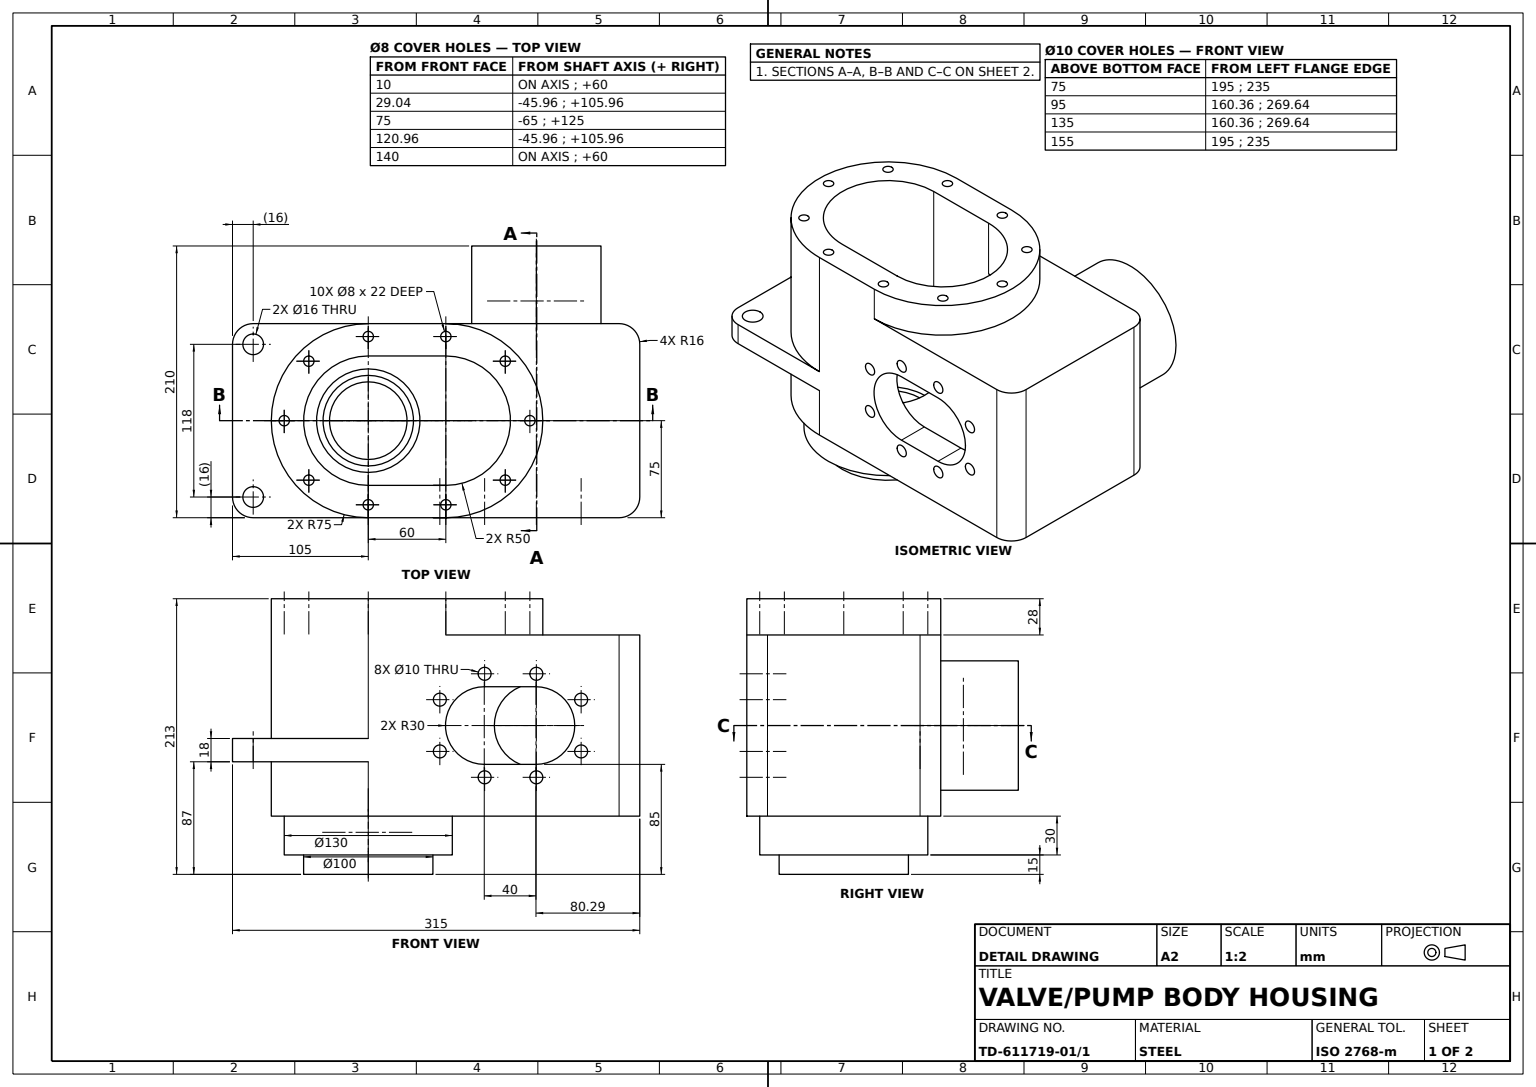
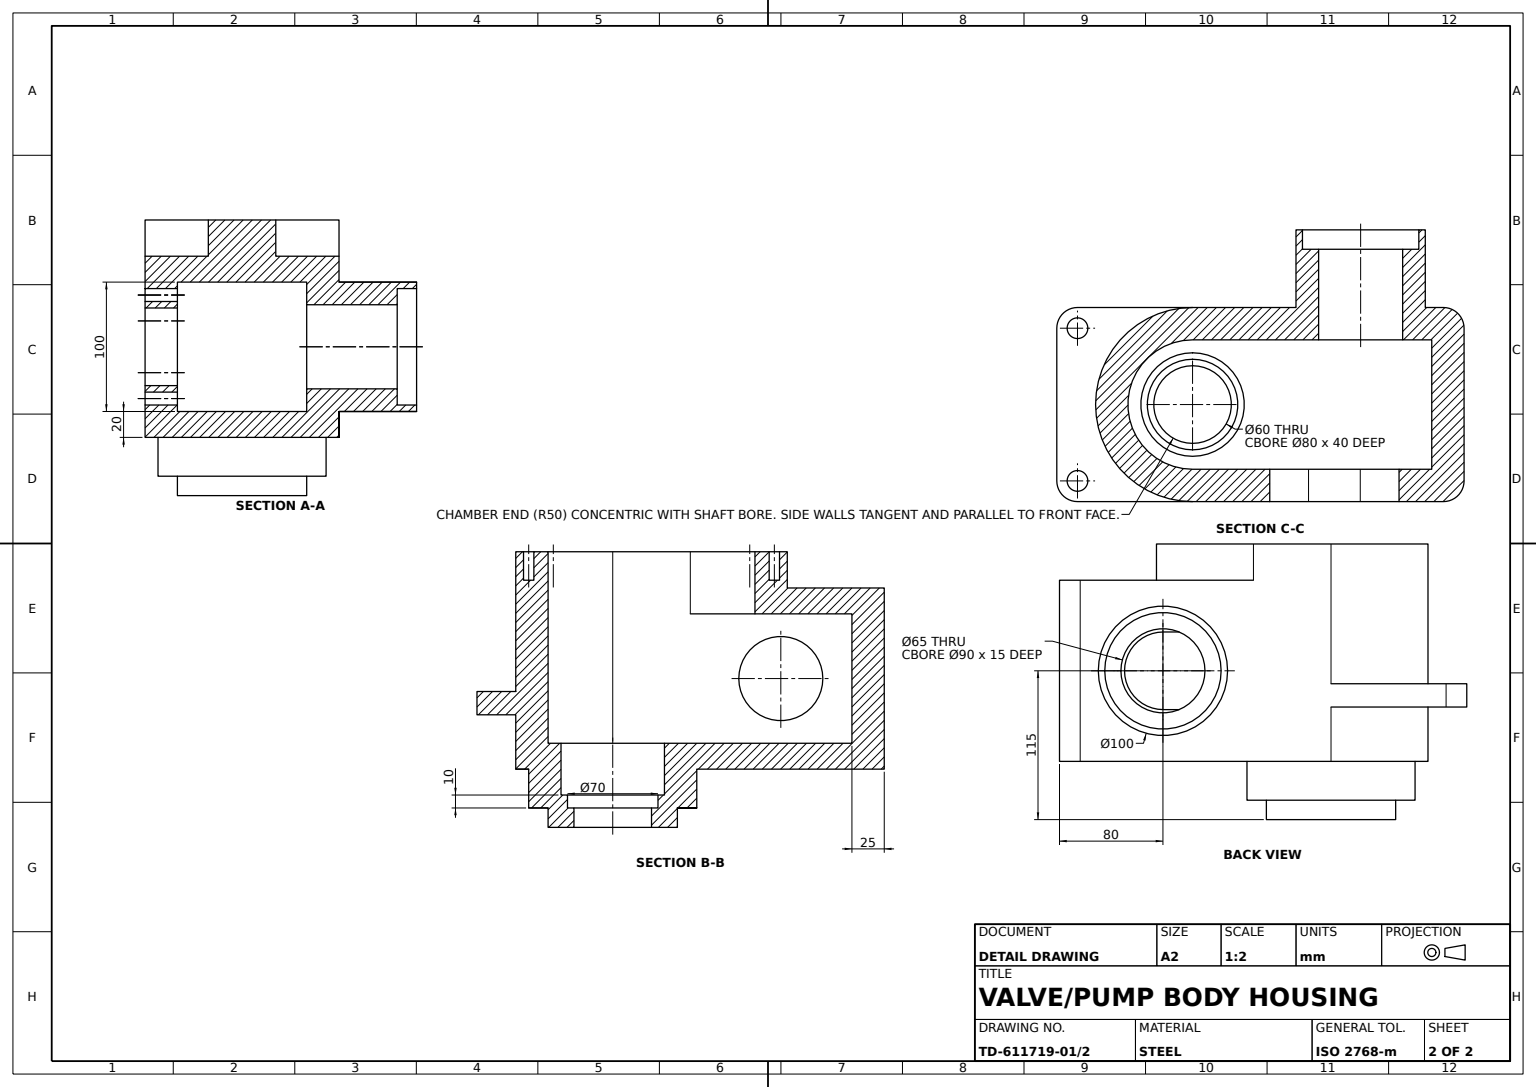
solid
v1 (0,213,61)
v2 (0,213,69)
e1 v1 v2 CIRCLE(AX(P(0,213,65),D(0,1,0),D(0,0,1)),4)
v3 (0,191,69)
e2 v3 v2 LINE
v4 (0,191,61)
e3 v4 v3 CIRCLE(AX(P(0,191,65),D(0,1,0),D(0,0,1)),4)
e4 v4 v1 LINE
face CYL(AX(P(0,191,65),D(0,1,0),D(0,0,1)),4) rev [e1 -e2 -e3 e4]
v5 (0,213,-75)
v6 (0,213,75)
e5 v5 v6 CIRCLE(AX(P(0,213,0),D(0,1,0),D(0,0,1)),75)
v7 (0,105,-75)
e6 v5 v7 LINE
v8 (0,105,75)
e7 v7 v8 CIRCLE(AX(P(0,105,0),D(0,1,0),D(0,0,-1)),75)
e8 v6 v8 LINE
face CYL(AX(P(0,213,0),D(0,-1,0),D(0,0,-1)),75) [-e5 e6 e7 -e8]
v9 (-105,87,59)
v10 (-105,105,59)
e9 v9 v10 LINE
v11 (-105,105,-59)
e10 v10 v11 LINE
v12 (-105,87,-59)
e11 v11 v12 LINE
e12 v9 v12 LINE
face PLANE(AX(P(-105,105,0),D(-1,0,0),D(0,0,1))) [e9 e10 e11 -e12]
v13 (129.708685,145,50)
v14 (129.708685,145,75)
e13 v13 v14 LINE
v15 (89.708685,145,75)
e14 v14 v15 LINE
v16 (89.708685,145,50)
e15 v16 v15 LINE
e16 v16 v13 LINE
face PLANE(AX(P(89.708685,145,-19),D(0,1,0),D(0,0,1))) rev [e13 e14 -e15 e16]
v17 (169.641016,135,50)
v18 (169.641016,135,75)
e17 v17 v18 LINE
v19 (159.641016,135,75)
e18 v18 v19 CIRCLE(AX(P(164.641016,135,75),D(0,0,1),D(1,0,0)),5)
v20 (159.641016,135,50)
e19 v20 v19 LINE
e20 v20 v17 CIRCLE(AX(P(164.641016,135,50),D(0,0,-1),D(1,0,0)),5)
face CYL(AX(P(164.641016,135,-19),D(0,0,1),D(1,0,0)),5) rev [e17 e18 -e19 e20]
v21 (125,191,-4)
v22 (125,191,4)
e21 v21 v22 CIRCLE(AX(P(125,191,0),D(0,1,0),D(0,0,1)),4)
e22 v22 v21 CIRCLE(AX(P(125,191,0),D(0,1,0),D(0,0,1)),4)
face PLANE(AX(P(125,191,0),D(0,1,0),D(0,0,1))) [e21 e22]
v23 (125,155,50)
v24 (135,155,50)
e23 v23 v24 CIRCLE(AX(P(130,155,50),D(0,0,-1),D(1,0,0)),5)
v25 (135,155,75)
e24 v24 v25 LINE
v26 (125,155,75)
e25 v25 v26 CIRCLE(AX(P(130,155,75),D(0,0,1),D(1,0,0)),5)
e26 v23 v26 LINE
face CYL(AX(P(130,155,-19),D(0,0,1),D(1,0,0)),5) rev [e23 e24 e25 -e26]
v27 (0,191,-69)
v28 (0,191,-61)
e27 v27 v28 CIRCLE(AX(P(0,191,-65),D(0,1,0),D(0,0,1)),4)
v29 (0,213,-69)
e28 v27 v29 LINE
v30 (0,213,-61)
e29 v29 v30 CIRCLE(AX(P(0,213,-65),D(0,1,0),D(0,0,1)),4)
e30 v28 v30 LINE
face CYL(AX(P(0,191,-65),D(0,1,0),D(0,0,1)),4) rev [-e27 e28 e29 -e30]
v31 (125,213,-4)
e31 v21 v31 LINE
v32 (125,213,4)
e32 v31 v32 CIRCLE(AX(P(125,213,0),D(0,1,0),D(0,0,1)),4)
e33 v22 v32 LINE
face CYL(AX(P(125,191,0),D(0,1,0),D(0,0,1)),4) rev [e31 e32 -e33 -e21]
v33 (0,25,-35)
v34 (0,25,35)
e34 v33 v34 CIRCLE(AX(P(0,25,0),D(0,-1,0),D(0,0,-1)),35)
e35 v34 v33 CIRCLE(AX(P(0,25,0),D(0,-1,0),D(0,0,-1)),35)
v35 (0,25,-40)
v36 (0,25,40)
e36 v35 v36 CIRCLE(AX(P(0,25,0),D(0,-1,0),D(0,0,-1)),40)
e37 v36 v35 CIRCLE(AX(P(0,25,0),D(0,-1,0),D(0,0,-1)),40)
face PLANE(AX(P(0,25,0),D(0,-1,0),D(0,0,-1))) rev [e34 e35] [-e36 -e37]
v37 (60,165,-50)
v38 (185,165,-50)
e38 v37 v38 LINE
v39 (185,165,50)
e39 v38 v39 LINE
v40 (60,165,50)
e40 v39 v40 LINE
e41 v37 v40 CIRCLE(AX(P(60,165,0),D(0,-1,0),D(0,0,-1)),50)
face PLANE(AX(P(0,165,0),D(0,-1,0),D(0,0,-1))) [e38 e39 e40 -e41]
v41 (60,191,-69)
v42 (60,191,-61)
e42 v41 v42 CIRCLE(AX(P(60,191,-65),D(0,1,0),D(0,0,1)),4)
e43 v42 v41 CIRCLE(AX(P(60,191,-65),D(0,1,0),D(0,0,1)),4)
face PLANE(AX(P(60,191,-65),D(0,1,0),D(0,0,1))) [e42 e43]
e44 v19 v18 CIRCLE(AX(P(164.641016,135,75),D(0,0,1),D(1,0,0)),5)
e45 v17 v20 CIRCLE(AX(P(164.641016,135,50),D(0,0,-1),D(1,0,0)),5)
face CYL(AX(P(164.641016,135,-19),D(0,0,1),D(1,0,0)),5) rev [e44 -e17 e45 e19]
v43 (-45.961941,191,49.961941)
v44 (-45.961941,213,49.961941)
e46 v43 v44 LINE
v45 (-45.961941,213,41.961941)
e47 v44 v45 CIRCLE(AX(P(-45.961941,213,45.961941),D(0,1,0),D(0,0,1)),4)
v46 (-45.961941,191,41.961941)
e48 v46 v45 LINE
e49 v43 v46 CIRCLE(AX(P(-45.961941,191,45.961941),D(0,1,0),D(0,0,1)),4)
face CYL(AX(P(-45.961941,191,45.961941),D(0,1,0),D(0,0,1)),4) rev [e46 e47 -e48 -e49]
v47 (105.961941,213,-41.961941)
v48 (105.961941,213,-49.961941)
e50 v47 v48 CIRCLE(AX(P(105.961941,213,-45.961941),D(0,1,0),D(0,0,1)),4)
v49 (105.961941,191,-49.961941)
e51 v49 v48 LINE
v50 (105.961941,191,-41.961941)
e52 v50 v49 CIRCLE(AX(P(105.961941,191,-45.961941),D(0,1,0),D(0,0,1)),4)
e53 v50 v47 LINE
face CYL(AX(P(105.961941,191,-45.961941),D(0,1,0),D(0,0,1)),4) rev [e50 -e51 -e52 e53]
v51 (159.641016,95,50)
v52 (159.641016,95,75)
e54 v51 v52 LINE
v53 (169.641016,95,75)
e55 v52 v53 CIRCLE(AX(P(164.641016,95,75),D(0,0,1),D(1,0,0)),5)
v54 (169.641016,95,50)
e56 v54 v53 LINE
e57 v54 v51 CIRCLE(AX(P(164.641016,95,50),D(0,0,-1),D(1,0,0)),5)
face CYL(AX(P(164.641016,95,-19),D(0,0,1),D(1,0,0)),5) rev [e54 e55 -e56 e57]
v55 (105.961941,191,49.961941)
v56 (105.961941,213,49.961941)
e58 v55 v56 LINE
v57 (105.961941,191,41.961941)
e59 v57 v55 CIRCLE(AX(P(105.961941,191,45.961941),D(0,1,0),D(0,0,1)),4)
v58 (105.961941,213,41.961941)
e60 v57 v58 LINE
e61 v58 v56 CIRCLE(AX(P(105.961941,213,45.961941),D(0,1,0),D(0,0,1)),4)
face CYL(AX(P(105.961941,191,45.961941),D(0,1,0),D(0,0,1)),4) rev [-e58 -e59 e60 e61]
e62 v49 v50 CIRCLE(AX(P(105.961941,191,-45.961941),D(0,1,0),D(0,0,1)),4)
e63 v48 v47 CIRCLE(AX(P(105.961941,213,-45.961941),D(0,1,0),D(0,0,1)),4)
face CYL(AX(P(105.961941,191,-45.961941),D(0,1,0),D(0,0,1)),4) rev [-e53 -e62 e51 e63]
v59 (-65,191,4)
v60 (-65,213,4)
e64 v59 v60 LINE
v61 (-65,213,-4)
e65 v60 v61 CIRCLE(AX(P(-65,213,0),D(0,1,0),D(0,0,1)),4)
v62 (-65,191,-4)
e66 v62 v61 LINE
e67 v59 v62 CIRCLE(AX(P(-65,191,0),D(0,1,0),D(0,0,1)),4)
face CYL(AX(P(-65,191,0),D(0,1,0),D(0,0,1)),4) rev [e64 e65 -e66 -e67]
v63 (0,45,75)
v64 (194,45,75)
e68 v63 v64 LINE
v65 (0,45,-75)
e69 v65 v63 CIRCLE(AX(P(0,45,0),D(0,1,0),D(0,0,1)),75)
v66 (194,45,-75)
e70 v66 v65 LINE
v67 (210,45,-59)
e71 v66 v67 CIRCLE(AX(P(194,45,-59),D(0,-1,0),D(0,0,1)),16)
v68 (210,45,59)
e72 v68 v67 LINE
e73 v68 v64 CIRCLE(AX(P(194,45,59),D(0,-1,0),D(0,0,1)),16)
v69 (0,45,-65)
v70 (0,45,65)
e74 v69 v70 CIRCLE(AX(P(0,45,0),D(0,1,0),D(0,0,1)),65)
e75 v70 v69 CIRCLE(AX(P(0,45,0),D(0,1,0),D(0,0,1)),65)
face PLANE(AX(P(0,45,0),D(0,1,0),D(0,0,1))) rev [-e68 -e69 -e70 e71 -e72 e73] [e74 e75]
v71 (0,15,65)
v72 (0,15,-65)
e76 v71 v72 CIRCLE(AX(P(0,15,0),D(0,1,0),D(0,0,1)),65)
e77 v72 v71 CIRCLE(AX(P(0,15,0),D(0,1,0),D(0,0,1)),65)
v73 (0,15,-50)
v74 (0,15,50)
e78 v73 v74 CIRCLE(AX(P(0,15,0),D(0,1,0),D(0,0,1)),50)
e79 v74 v73 CIRCLE(AX(P(0,15,0),D(0,1,0),D(0,0,1)),50)
face PLANE(AX(P(0,15,0),D(0,1,0),D(0,0,1))) rev [-e76 -e77] [e78 e79]
v75 (0,15,30)
v76 (0,15,-30)
e80 v75 v76 CIRCLE(AX(P(0,15,0),D(0,-1,0),D(0,0,-1)),30)
v77 (0,0,30)
e81 v75 v77 LINE
v78 (0,0,-30)
e82 v77 v78 CIRCLE(AX(P(0,0,0),D(0,-1,0),D(0,0,-1)),30)
e83 v76 v78 LINE
face CYL(AX(P(0,15,0),D(0,-1,0),D(0,0,-1)),30) rev [-e80 e81 e82 -e83]
e84 v70 v71 LINE
e85 v69 v72 LINE
face CYL(AX(P(0,45,0),D(0,-1,0),D(0,0,-1)),65) [-e75 e84 e76 -e85]
e86 v62 v59 CIRCLE(AX(P(-65,191,0),D(0,1,0),D(0,0,1)),4)
face PLANE(AX(P(-65,191,0),D(0,1,0),D(0,0,1))) [e67 e86]
v79 (60,213,-69)
v80 (60,213,-61)
e87 v79 v80 CIRCLE(AX(P(60,213,-65),D(0,1,0),D(0,0,1)),4)
e88 v80 v79 CIRCLE(AX(P(60,213,-65),D(0,1,0),D(0,0,1)),4)
e89 v61 v60 CIRCLE(AX(P(-65,213,0),D(0,1,0),D(0,0,1)),4)
e90 v56 v58 CIRCLE(AX(P(105.961941,213,45.961941),D(0,1,0),D(0,0,1)),4)
e91 v32 v31 CIRCLE(AX(P(125,213,0),D(0,1,0),D(0,0,1)),4)
e92 v45 v44 CIRCLE(AX(P(-45.961941,213,45.961941),D(0,1,0),D(0,0,1)),4)
v81 (60,213,69)
v82 (60,213,61)
e93 v81 v82 CIRCLE(AX(P(60,213,65),D(0,1,0),D(0,0,1)),4)
e94 v82 v81 CIRCLE(AX(P(60,213,65),D(0,1,0),D(0,0,1)),4)
e95 v2 v1 CIRCLE(AX(P(0,213,65),D(0,1,0),D(0,0,1)),4)
v83 (-45.961941,213,-41.961941)
v84 (-45.961941,213,-49.961941)
e96 v83 v84 CIRCLE(AX(P(-45.961941,213,-45.961941),D(0,1,0),D(0,0,1)),4)
e97 v84 v83 CIRCLE(AX(P(-45.961941,213,-45.961941),D(0,1,0),D(0,0,1)),4)
v85 (0,213,-50)
v86 (0,213,50)
e98 v85 v86 CIRCLE(AX(P(0,213,0),D(0,1,0),D(0,0,1)),50)
v87 (60,213,-50)
e99 v87 v85 LINE
v88 (60,213,50)
e100 v88 v87 CIRCLE(AX(P(60,213,0),D(0,1,0),D(0,0,1)),50)
e101 v86 v88 LINE
v89 (60,213,75)
e102 v6 v89 LINE
v90 (60,213,-75)
e103 v90 v89 CIRCLE(AX(P(60,213,0),D(0,-1,0),D(0,0,1)),75)
e104 v90 v5 LINE
e105 v30 v29 CIRCLE(AX(P(0,213,-65),D(0,1,0),D(0,0,1)),4)
face PLANE(AX(P(0,213,0),D(0,1,0),D(0,0,1))) [-e87 -e88] [-e65 -e89] [-e90 -e61] [-e32 -e91] [-e47 -e92] [-e93 -e94] [-e1 -e95] [-e50 -e63] [-e96 -e97] [-e98 -e99 -e100 -e101] [e102 -e103 e104 e5] [-e105 -e29]
v91 (0,0,50)
e106 v74 v91 LINE
v92 (0,0,-50)
e107 v91 v92 CIRCLE(AX(P(0,0,0),D(0,1,0),D(0,0,1)),50)
e108 v73 v92 LINE
face CYL(AX(P(0,15,0),D(0,-1,0),D(0,0,-1)),50) [-e79 e106 e107 -e108]
v93 (89.708685,85,75)
e109 v15 v93 CIRCLE(AX(P(89.708685,115,75),D(0,0,1),D(1,0,0)),30)
v94 (89.708685,85,50)
e110 v94 v93 LINE
e111 v94 v16 CIRCLE(AX(P(89.708685,115,50),D(0,0,-1),D(1,0,0)),30)
face CYL(AX(P(89.708685,115,-19),D(0,0,1),D(1,0,0)),30) rev [e15 e109 -e110 e111]
e112 v42 v80 LINE
e113 v41 v79 LINE
face CYL(AX(P(60,191,-65),D(0,1,0),D(0,0,1)),4) rev [-e43 e112 e88 -e113]
v95 (85,115,-120)
v96 (85,115,-135)
e114 v95 v96 LINE
v97 (175,115,-120)
e115 v97 v95 CIRCLE(AX(P(130,115,-120),D(0,0,-1),D(-1,0,0)),45)
v98 (175,115,-135)
e116 v97 v98 LINE
e117 v98 v96 CIRCLE(AX(P(130,115,-135),D(0,0,-1),D(-1,0,0)),45)
face CYL(AX(P(130,115,-120),D(0,0,-1),D(-1,0,0)),45) rev [-e114 -e115 e116 e117]
face CYL(AX(P(60,191,-65),D(0,1,0),D(0,0,1)),4) rev [-e42 e113 e87 -e112]
v99 (85,75,50)
v100 (95,75,50)
e118 v99 v100 CIRCLE(AX(P(90,75,50),D(0,0,-1),D(1,0,0)),5)
v101 (95,75,75)
e119 v100 v101 LINE
v102 (85,75,75)
e120 v101 v102 CIRCLE(AX(P(90,75,75),D(0,0,1),D(1,0,0)),5)
e121 v99 v102 LINE
face CYL(AX(P(90,75,-19),D(0,0,1),D(1,0,0)),5) rev [e118 e119 e120 -e121]
v103 (95,155,75)
v104 (85,155,75)
e122 v103 v104 CIRCLE(AX(P(90,155,75),D(0,0,1),D(1,0,0)),5)
v105 (85,155,50)
e123 v105 v104 LINE
v106 (95,155,50)
e124 v105 v106 CIRCLE(AX(P(90,155,50),D(0,0,-1),D(1,0,0)),5)
e125 v106 v103 LINE
face CYL(AX(P(90,155,-19),D(0,0,1),D(1,0,0)),5) rev [e122 -e123 e124 e125]
v107 (0,65,-40)
e126 v107 v35 LINE
v108 (0,65,40)
e127 v108 v107 CIRCLE(AX(P(0,65,0),D(0,-1,0),D(0,0,-1)),40)
e128 v108 v36 LINE
face CYL(AX(P(0,144,0),D(0,-1,0),D(0,0,-1)),40) rev [e37 -e126 -e127 e128]
e129 v76 v75 CIRCLE(AX(P(0,15,0),D(0,-1,0),D(0,0,-1)),30)
v109 (0,15,-35)
v110 (0,15,35)
e130 v109 v110 CIRCLE(AX(P(0,15,0),D(0,-1,0),D(0,0,-1)),35)
e131 v110 v109 CIRCLE(AX(P(0,15,0),D(0,-1,0),D(0,0,-1)),35)
face PLANE(AX(P(0,15,0),D(0,-1,0),D(0,0,-1))) rev [e80 e129] [-e130 -e131]
e132 v34 v110 LINE
e133 v33 v109 LINE
face CYL(AX(P(0,25,0),D(0,-1,0),D(0,0,-1)),35) rev [-e132 -e34 e133 e130]
e134 v40 v88 LINE
e135 v37 v87 LINE
face CYL(AX(P(60,122,0),D(0,1,0),D(0,0,1)),50) rev [e134 e100 -e135 e41]
v111 (60.358984,135,50)
v112 (60.358984,135,75)
e136 v111 v112 LINE
v113 (50.358984,135,50)
e137 v111 v113 CIRCLE(AX(P(55.358984,135,50),D(0,0,-1),D(1,0,0)),5)
v114 (50.358984,135,75)
e138 v113 v114 LINE
e139 v114 v112 CIRCLE(AX(P(55.358984,135,75),D(0,0,1),D(1,0,0)),5)
face CYL(AX(P(55.358984,135,-19),D(0,0,1),D(1,0,0)),5) rev [-e136 e137 e138 e139]
e140 v107 v108 CIRCLE(AX(P(0,65,0),D(0,-1,0),D(0,0,-1)),40)
face CYL(AX(P(0,144,0),D(0,-1,0),D(0,0,-1)),40) rev [e36 -e128 -e140 e126]
e141 v78 v77 CIRCLE(AX(P(0,0,0),D(0,-1,0),D(0,0,-1)),30)
e142 v92 v91 CIRCLE(AX(P(0,0,0),D(0,1,0),D(0,0,1)),50)
face PLANE(AX(P(0,0,0),D(0,1,0),D(0,0,1))) rev [-e141 -e82] [-e107 -e142]
face CYL(AX(P(0,15,0),D(0,-1,0),D(0,0,-1)),30) rev [e83 e141 -e81 -e129]
v115 (210,185,59)
e143 v115 v68 LINE
v116 (194,185,75)
e144 v116 v115 CIRCLE(AX(P(194,185,59),D(0,1,0),D(0,0,1)),16)
e145 v64 v116 LINE
face CYL(AX(P(194,213,59),D(0,-1,0),D(0,0,-1)),16) [-e143 -e144 -e145 -e73]
v117 (210,185,-59)
e146 v67 v117 LINE
e147 v115 v117 LINE
face PLANE(AX(P(210,213,75),D(-1,0,0),D(0,0,1))) rev [e72 e146 -e147 e143]
v118 (80,115,-135)
v119 (180,115,-135)
e148 v118 v119 CIRCLE(AX(P(130,115,-135),D(0,0,-1),D(-1,0,0)),50)
e149 v119 v118 CIRCLE(AX(P(130,115,-135),D(0,0,-1),D(-1,0,0)),50)
e150 v96 v98 CIRCLE(AX(P(130,115,-135),D(0,0,-1),D(-1,0,0)),45)
face PLANE(AX(P(130,115,-135),D(0,0,-1),D(-1,0,0))) [e148 e149] [-e117 -e150]
v120 (180,115,-75)
e151 v119 v120 LINE
v121 (80,115,-75)
e152 v118 v121 LINE
e153 v121 v120 CIRCLE(AX(P(130,115,-75),D(0,0,-1),D(1,0,0)),50)
face CYL(AX(P(130,115,-135),D(0,0,1),D(1,0,0)),50) [-e151 -e148 e152 e153]
e154 v51 v54 CIRCLE(AX(P(164.641016,95,50),D(0,0,-1),D(1,0,0)),5)
v122 (185,65,50)
e155 v39 v122 LINE
v123 (0,65,50)
e156 v122 v123 LINE
e157 v86 v123 LINE
v124 (159.708685,115,50)
v125 (129.708685,85,50)
e158 v124 v125 CIRCLE(AX(P(129.708685,115,50),D(0,0,-1),D(1,0,0)),30)
e159 v13 v124 CIRCLE(AX(P(129.708685,115,50),D(0,0,-1),D(1,0,0)),30)
e160 v125 v94 LINE
e161 v106 v105 CIRCLE(AX(P(90,155,50),D(0,0,-1),D(1,0,0)),5)
e162 v100 v99 CIRCLE(AX(P(90,75,50),D(0,0,-1),D(1,0,0)),5)
e163 v24 v23 CIRCLE(AX(P(130,155,50),D(0,0,-1),D(1,0,0)),5)
v126 (50.358984,95,50)
v127 (60.358984,95,50)
e164 v126 v127 CIRCLE(AX(P(55.358984,95,50),D(0,0,-1),D(1,0,0)),5)
e165 v127 v126 CIRCLE(AX(P(55.358984,95,50),D(0,0,-1),D(1,0,0)),5)
e166 v113 v111 CIRCLE(AX(P(55.358984,135,50),D(0,0,-1),D(1,0,0)),5)
v128 (125,75,50)
v129 (135,75,50)
e167 v128 v129 CIRCLE(AX(P(130,75,50),D(0,0,-1),D(1,0,0)),5)
e168 v129 v128 CIRCLE(AX(P(130,75,50),D(0,0,-1),D(1,0,0)),5)
face PLANE(AX(P(185,165,50),D(0,0,1),D(1,0,0))) rev [-e57 -e154] [e155 e156 -e157 e101 -e134 -e40] [-e158 -e159 -e16 -e111 -e160] [-e20 -e45] [-e161 -e124] [-e162 -e118] [-e163 -e23] [-e164 -e165] [-e166 -e137] [-e167 -e168]
v130 (-89,87,75)
e169 v130 v9 CIRCLE(AX(P(-89,87,59),D(0,-1,0),D(0,0,-1)),16)
v131 (-89,105,75)
e170 v131 v130 LINE
e171 v10 v131 CIRCLE(AX(P(-89,105,59),D(0,1,0),D(0,0,-1)),16)
face CYL(AX(P(-89,213,59),D(0,1,0),D(0,0,1)),16) [-e169 -e170 -e171 -e9]
v132 (129.708685,85,75)
e172 v125 v132 LINE
v133 (159.708685,115,75)
e173 v132 v133 CIRCLE(AX(P(129.708685,115,75),D(0,0,1),D(1,0,0)),30)
e174 v124 v133 LINE
face CYL(AX(P(129.708685,115,-19),D(0,0,1),D(1,0,0)),30) rev [e158 e172 e173 -e174]
e175 v53 v52 CIRCLE(AX(P(164.641016,95,75),D(0,0,1),D(1,0,0)),5)
face CYL(AX(P(164.641016,95,-19),D(0,0,1),D(1,0,0)),5) rev [e154 e56 e175 -e54]
v134 (125,75,75)
v135 (135,75,75)
e176 v134 v135 CIRCLE(AX(P(130,75,75),D(0,0,1),D(1,0,0)),5)
e177 v129 v135 LINE
e178 v128 v134 LINE
face CYL(AX(P(130,75,-19),D(0,0,1),D(1,0,0)),5) rev [e176 -e177 e168 e178]
e179 v55 v57 CIRCLE(AX(P(105.961941,191,45.961941),D(0,1,0),D(0,0,1)),4)
face PLANE(AX(P(105.961941,191,45.961941),D(0,1,0),D(0,0,1))) [e179 e59]
v136 (-45.961941,191,-49.961941)
e180 v136 v84 LINE
v137 (-45.961941,191,-41.961941)
e181 v137 v83 LINE
e182 v136 v137 CIRCLE(AX(P(-45.961941,191,-45.961941),D(0,1,0),D(0,0,1)),4)
face CYL(AX(P(-45.961941,191,-45.961941),D(0,1,0),D(0,0,1)),4) rev [e180 e97 -e181 -e182]
e183 v137 v136 CIRCLE(AX(P(-45.961941,191,-45.961941),D(0,1,0),D(0,0,1)),4)
face CYL(AX(P(-45.961941,191,-45.961941),D(0,1,0),D(0,0,1)),4) rev [-e180 -e183 e181 e96]
v138 (50.358984,95,75)
e184 v126 v138 LINE
v139 (60.358984,95,75)
e185 v138 v139 CIRCLE(AX(P(55.358984,95,75),D(0,0,1),D(1,0,0)),5)
e186 v127 v139 LINE
face CYL(AX(P(55.358984,95,-19),D(0,0,1),D(1,0,0)),5) rev [e165 e184 e185 -e186]
v140 (-89,105,-75)
e187 v140 v11 CIRCLE(AX(P(-89,105,-59),D(0,1,0),D(0,0,-1)),16)
v141 (-89,87,-75)
e188 v141 v140 LINE
e189 v12 v141 CIRCLE(AX(P(-89,87,-59),D(0,-1,0),D(0,0,-1)),16)
face CYL(AX(P(-89,105,-59),D(0,1,0),D(0,0,1)),16) [-e187 -e188 -e189 -e11]
e190 v28 v27 CIRCLE(AX(P(0,191,-65),D(0,1,0),D(0,0,1)),4)
face CYL(AX(P(0,191,-65),D(0,1,0),D(0,0,1)),4) rev [-e190 e30 e105 -e28]
face PLANE(AX(P(-45.961941,191,-45.961941),D(0,1,0),D(0,0,1))) [e182 e183]
e191 v95 v97 CIRCLE(AX(P(130,115,-120),D(0,0,-1),D(-1,0,0)),45)
face CYL(AX(P(130,115,-120),D(0,0,-1),D(-1,0,0)),45) rev [e114 e150 -e116 -e191]
face CYL(AX(P(105.961941,191,45.961941),D(0,1,0),D(0,0,1)),4) rev [-e179 e58 e90 -e60]
e192 v3 v4 CIRCLE(AX(P(0,191,65),D(0,1,0),D(0,0,1)),4)
face CYL(AX(P(0,191,65),D(0,1,0),D(0,0,1)),4) rev [-e192 e2 e95 -e4]
e193 v135 v134 CIRCLE(AX(P(130,75,75),D(0,0,1),D(1,0,0)),5)
face CYL(AX(P(130,75,-19),D(0,0,1),D(1,0,0)),5) rev [e167 e177 e193 -e178]
v142 (-89,105,67)
v143 (-89,105,51)
e194 v142 v143 CIRCLE(AX(P(-89,105,59),D(0,1,0),D(0,0,1)),8)
v144 (-89,87,51)
e195 v144 v143 LINE
v145 (-89,87,67)
e196 v144 v145 CIRCLE(AX(P(-89,87,59),D(0,-1,0),D(0,0,-1)),8)
e197 v145 v142 LINE
face CYL(AX(P(-89,14,59),D(0,1,0),D(0,0,1)),8) rev [e194 -e195 e196 e197]
v146 (0,65,-50)
e198 v123 v146 CIRCLE(AX(P(0,65,0),D(0,-1,0),D(0,0,-1)),50)
v147 (185,65,-50)
e199 v147 v122 LINE
e200 v146 v147 LINE
face PLANE(AX(P(0,65,0),D(0,-1,0),D(0,0,-1))) rev [-e198 -e156 -e199 -e200] [e127 e140]
e201 v112 v114 CIRCLE(AX(P(55.358984,135,75),D(0,0,1),D(1,0,0)),5)
face CYL(AX(P(55.358984,135,-19),D(0,0,1),D(1,0,0)),5) rev [e136 e201 -e138 e166]
e202 v38 v147 LINE
face PLANE(AX(P(185,165,-50),D(1,0,0),D(0,0,-1))) rev [e202 e199 -e155 -e39]
e203 v26 v25 CIRCLE(AX(P(130,155,75),D(0,0,1),D(1,0,0)),5)
e204 v93 v132 LINE
e205 v133 v14 CIRCLE(AX(P(129.708685,115,75),D(0,0,1),D(1,0,0)),30)
e206 v139 v138 CIRCLE(AX(P(55.358984,95,75),D(0,0,1),D(1,0,0)),5)
e207 v104 v103 CIRCLE(AX(P(90,155,75),D(0,0,1),D(1,0,0)),5)
e208 v102 v101 CIRCLE(AX(P(90,75,75),D(0,0,1),D(1,0,0)),5)
v148 (0,87,75)
e209 v148 v63 LINE
v149 (60,185,75)
e210 v149 v116 LINE
e211 v149 v89 LINE
e212 v8 v131 LINE
e213 v148 v130 LINE
face PLANE(AX(P(0,213,75),D(0,0,-1),D(-1,0,0))) rev [-e203 -e25] [-e173 -e204 -e109 -e14 -e205] [-e206 -e185] [-e44 -e18] [-e122 -e207] [-e139 -e201] [-e193 -e176] [-e120 -e208] [e209 e68 e145 -e210 e211 -e102 e8 e212 e170 -e213] [-e55 -e175]
v150 (-89,87,-67)
v151 (-89,87,-51)
e214 v150 v151 CIRCLE(AX(P(-89,87,-59),D(0,-1,0),D(0,0,-1)),8)
v152 (-89,105,-51)
e215 v151 v152 LINE
v153 (-89,105,-67)
e216 v152 v153 CIRCLE(AX(P(-89,105,-59),D(0,1,0),D(0,0,1)),8)
e217 v150 v153 LINE
face CYL(AX(P(-89,14,-59),D(0,1,0),D(0,0,1)),8) rev [e214 e215 e216 -e217]
face CYL(AX(P(0,15,0),D(0,-1,0),D(0,0,-1)),50) [-e78 e108 e142 -e106]
v154 (194,185,-75)
e218 v154 v66 LINE
e219 v117 v154 CIRCLE(AX(P(194,185,-59),D(0,1,0),D(0,0,1)),16)
face CYL(AX(P(194,213,-59),D(0,-1,0),D(0,0,-1)),16) [-e71 -e218 -e219 -e146]
face CYL(AX(P(130,155,-19),D(0,0,1),D(1,0,0)),5) rev [e163 e26 e203 -e24]
face CYL(AX(P(0,45,0),D(0,-1,0),D(0,0,-1)),65) [-e84 -e74 e85 e77]
e220 v151 v150 CIRCLE(AX(P(-89,87,-59),D(0,-1,0),D(0,0,-1)),8)
e221 v153 v152 CIRCLE(AX(P(-89,105,-59),D(0,1,0),D(0,0,1)),8)
face CYL(AX(P(-89,14,-59),D(0,1,0),D(0,0,1)),8) rev [-e215 e220 e217 e221]
e222 v143 v142 CIRCLE(AX(P(-89,105,59),D(0,1,0),D(0,0,1)),8)
e223 v140 v7 LINE
face PLANE(AX(P(0,105,0),D(0,-1,0),D(0,0,-1))) rev [-e222 -e194] [-e221 -e216] [e187 -e10 e171 -e212 -e7 -e223]
face PLANE(AX(P(89.708685,85,-19),D(0,-1,0),D(0,0,-1))) rev [-e172 e160 e110 e204]
v155 (97.5,115,-50)
v156 (162.5,115,-50)
e224 v155 v156 CIRCLE(AX(P(130,115,-50),D(0,0,1),D(-1,0,0)),32.5)
e225 v156 v155 CIRCLE(AX(P(130,115,-50),D(0,0,1),D(-1,0,0)),32.5)
e226 v85 v146 LINE
face PLANE(AX(P(0,165,-50),D(0,0,-1),D(-1,0,0))) rev [-e224 -e225] [-e202 -e38 e135 e99 e226 e200]
face CYL(AX(P(-65,191,0),D(0,1,0),D(0,0,1)),4) rev [-e64 -e86 e66 e89]
face CYL(AX(P(55.358984,95,-19),D(0,0,1),D(1,0,0)),5) rev [e206 -e184 e164 e186]
face CYL(AX(P(90,75,-19),D(0,0,1),D(1,0,0)),5) rev [e162 e121 e208 -e119]
v157 (97.5,115,-120)
v158 (162.5,115,-120)
e227 v157 v158 CIRCLE(AX(P(130,115,-120),D(0,0,-1),D(-1,0,0)),32.5)
e228 v158 v157 CIRCLE(AX(P(130,115,-120),D(0,0,-1),D(-1,0,0)),32.5)
face PLANE(AX(P(130,115,-120),D(0,0,-1),D(-1,0,0))) [-e227 -e228] [e191 e115]
face CYL(AX(P(125,191,0),D(0,1,0),D(0,0,1)),4) rev [e91 -e31 -e22 e33]
e229 v46 v43 CIRCLE(AX(P(-45.961941,191,45.961941),D(0,1,0),D(0,0,1)),4)
face CYL(AX(P(-45.961941,191,45.961941),D(0,1,0),D(0,0,1)),4) rev [-e229 e48 e92 -e46]
v159 (60,191,69)
v160 (60,191,61)
e230 v159 v160 CIRCLE(AX(P(60,191,65),D(0,1,0),D(0,0,1)),4)
e231 v159 v81 LINE
e232 v160 v82 LINE
face CYL(AX(P(60,191,65),D(0,1,0),D(0,0,1)),4) rev [-e230 e231 e93 -e232]
face CYL(AX(P(0,25,0),D(0,-1,0),D(0,0,-1)),35) rev [-e35 e132 e131 -e133]
e233 v160 v159 CIRCLE(AX(P(60,191,65),D(0,1,0),D(0,0,1)),4)
face PLANE(AX(P(60,191,65),D(0,1,0),D(0,0,1))) [e230 e233]
e234 v120 v121 CIRCLE(AX(P(130,115,-75),D(0,0,-1),D(1,0,0)),50)
face CYL(AX(P(130,115,-135),D(0,0,1),D(1,0,0)),50) [e234 -e152 -e149 e151]
face PLANE(AX(P(105.961941,191,-45.961941),D(0,1,0),D(0,0,1))) [e62 e52]
face CYL(AX(P(0,165,0),D(0,-1,0),D(0,0,-1)),50) rev [-e226 e98 e157 e198]
e235 v156 v158 LINE
e236 v155 v157 LINE
face CYL(AX(P(130,115,30),D(0,0,-1),D(-1,0,0)),32.5) rev [e235 e228 -e236 e224]
face CYL(AX(P(130,115,30),D(0,0,-1),D(-1,0,0)),32.5) rev [e225 e236 e227 -e235]
face PLANE(AX(P(0,191,65),D(0,1,0),D(0,0,1))) [e192 e3]
v161 (60,185,-75)
e237 v161 v90 LINE
e238 v154 v161 LINE
v162 (0,87,-75)
e239 v162 v65 LINE
e240 v141 v162 LINE
face PLANE(AX(P(210,213,-75),D(0,0,1),D(1,0,0))) rev [-e234 -e153] [-e237 -e238 e218 e70 -e239 -e240 e188 e223 -e6 -e104]
face CYL(AX(P(60,191,65),D(0,1,0),D(0,0,1)),4) rev [-e231 -e233 e232 e94]
e241 v161 v149 CIRCLE(AX(P(60,185,0),D(0,-1,0),D(0,0,1)),75)
face PLANE(AX(P(60,185,0),D(0,1,0),D(0,0,1))) [e219 e238 e241 e210 e144 e147]
face PLANE(AX(P(-45.961941,191,45.961941),D(0,1,0),D(0,0,1))) [e49 e229]
e242 v145 v144 CIRCLE(AX(P(-89,87,59),D(0,-1,0),D(0,0,-1)),8)
face CYL(AX(P(-89,14,59),D(0,1,0),D(0,0,1)),8) rev [-e197 e242 e195 e222]
e243 v162 v148 CIRCLE(AX(P(0,87,0),D(0,1,0),D(0,0,-1)),75)
face CYL(AX(P(0,213,0),D(0,-1,0),D(0,0,-1)),75) [e239 e69 -e209 -e243]
face PLANE(AX(P(0,87,0),D(0,-1,0),D(0,0,-1))) [e213 e169 e12 e189 e240 e243] [-e220 -e214] [-e242 -e196]
face CYL(AX(P(60,185,0),D(0,1,0),D(0,0,1)),75) [e103 -e211 -e241 e237]
face CYL(AX(P(129.708685,115,-19),D(0,0,1),D(1,0,0)),30) rev [-e13 e159 e174 e205]
face PLANE(AX(P(0,191,-65),D(0,1,0),D(0,0,1))) [e27 e190]
face CYL(AX(P(90,155,-19),D(0,0,1),D(1,0,0)),5) rev [e161 e123 e207 -e125]
